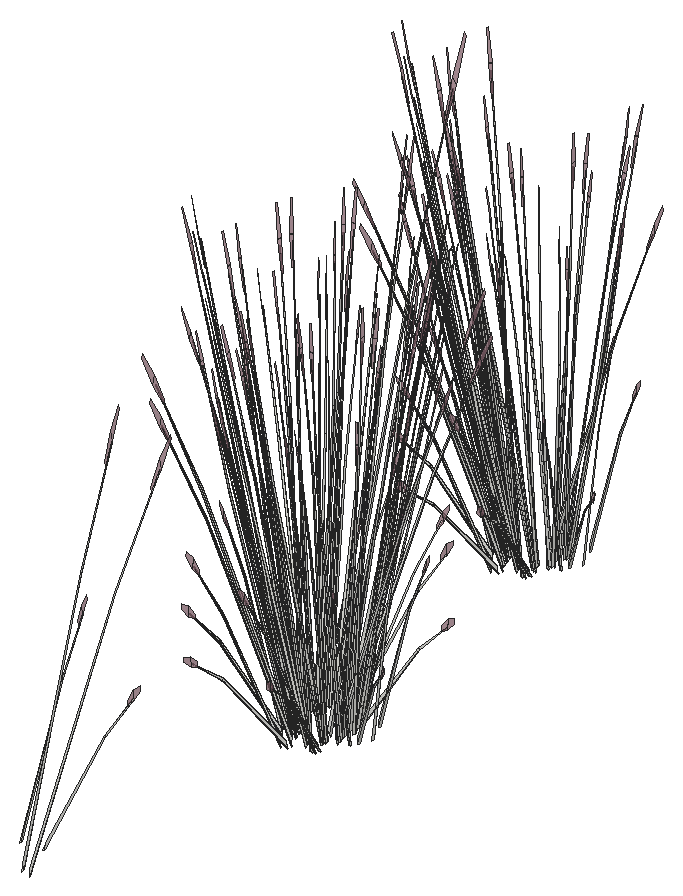
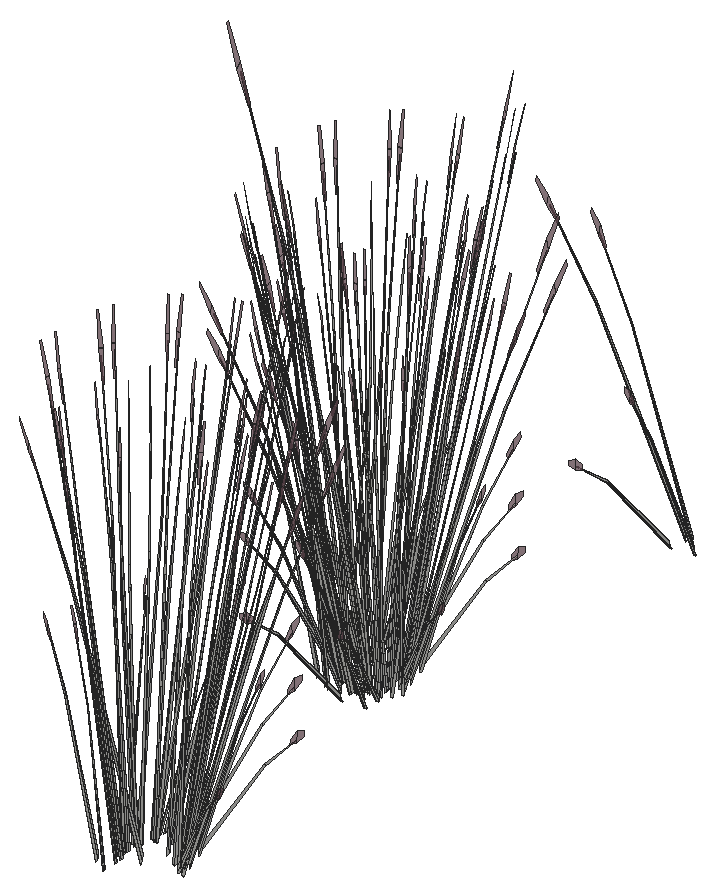
# SketchUp Ruby script. Lengths in inches.
U = 1.inch
M = Sketchup.active_model
def pt(a) = Geom::Point3d.new(a.map { |v| v * U })
def face(e, loops, mat)
  f = e.add_face(loops[0].map { |a| pt(a) })
  loops[1..].each { |l| e.add_face(l.map { |a| pt(a) }).erase! }
  f.material = f.back_material = mat if mat
  f
end
# faces: each face lists its corners as indices into pts; further lists are holes
def faces(e, pts, list, mat = nil) = list.each { |f| face(e, (f[0].is_a?(Array) ? f : [f]).map { |l| l.map { |i| pts[i] } }, mat) }
# xy, xz, yz: faces in a plane at the given z, y or x. An outline is a flat list of corners, or four numbers for a rectangle; further outlines are holes
def ring(l) = l.size == 4 ? [[l[0], l[1]], [l[2], l[1]], [l[2], l[3]], [l[0], l[3]]] : l.each_slice(2).to_a
def flat(e, list, mat, &to3) = list.each { |f| face(e, (f[0].is_a?(Array) ? f : [f]).map { |l| ring(l).map { |u, v| to3.(u, v) } }, mat) }
def xy(e, z, list, mat = nil) = flat(e, list, mat) { |x, y| [x, y, z] }
def xz(e, y, list, mat = nil) = flat(e, list, mat) { |x, z| [x, y, z] }
def yz(e, x, list, mat = nil) = flat(e, list, mat) { |y, z| [x, y, z] }
def lines(e, pts, list) = list.each { |a, b| e.add_line(pt(pts[a]), pt(pts[b])) }
# prism: a flat outline (further loops are holes) pulled along v
def prism(e, loops, v, mat = nil)
  f = face(e, loops, mat); d = Geom::Vector3d.new(v.map { |x| x * U })
  f.pushpull(f.normal.samedirection?(d) ? d.length : -d.length)
end
def box(e, o, s, mat = nil) = prism(e, [[o, [o[0] + s[0], o[1], o[2]], [o[0] + s[0], o[1] + s[1], o[2]], [o[0], o[1] + s[1], o[2]]]], [0, 0, s[2]], mat)
def at(x, y, z, deg = 0) = Geom::Transformation.translation(pt([x, y, z])) * Geom::Transformation.rotation(ORIGIN, Z_AXIS, deg.degrees)
def axes(o, x, y, z) = Geom::Transformation.new([*x, 0, *y, 0, *z, 0, *pt(o).to_a, 1])
def part(name) = M.definitions.add(name)
# library, detail: a bought-in or finely detailed component or shape, given as its bounding box
def library(name, o, s) = part(name).tap { |d| box(d.entities, o, s) }
def detail(e, o, s) = box(e.add_group.entities, o, s)
def put(e, d, t, mat = nil) = e.add_instance(d, t).tap { |i| i.material = mat if mat }
def group(e, t, mat = nil) = e.add_group.tap { |g| g.transformation = t; g.material = mat if mat }.entities
root = M.entities
M.materials.add("LightPink_Translucent").color = [144, 107, 117]
M.materials["LightPink_Translucent"].alpha = 0.75
c1 = part("blade")
p = [[2.15,0.21,22],[0,0.17,0],[0.09,0.45,0],[2.18,0.31,22],[2.29,0.31,22],[0.38,0.45,0],
  [2.48,0.24,33],[2.49,0.24,33],[2.48,0.22,33]]
faces(c1.entities,p,[[0,1,2,3],[4,5,2,3],[6,3,4,7],[8,0,3,6]])
c2 = part("seeds")
p = [[0.3,-0.1,1.38],[-0.01,-0.03,1.59],[-0.01,-0.03,0.03],[0.14,-0.07,-0.07],[0.29,-0.03,3],[0.15,0.01,3.11]]
faces(c2.entities,p,[[0,1,2,3],[1,0,4,5]],"LightPink_Translucent")
c3 = part("blade with seeds")
put(c3.entities,c1,at(0,0,0))
put(c3.entities,c2,axes([2.4,0.25,30.99],[1.5799,-0.05474,1.17369],[-0.12525,1.92788,0.29478],[-0.07173,-0.02425,1.56792]))
put(root,c3,axes([432.62,162.45,1.33],[-0.08601,-0.17716,1.47384],[0.39746,-0.14915,0.11917],[0.08983,0.27813,0.63005]))
put(root,c3,axes([430.45,164.24,2.05],[0.04269,-0.03331,1.5255],[0.35284,0.2216,-0.14414],[-0.00829,0.1845,0.26996]))
put(root,c3,axes([431.92,162.54,1.33],[-0.00921,-0.21179,1.47384],[0.39917,0.1405,0.11917],[-0.02469,0.30182,0.63005]))
put(root,c3,axes([432.01,164.47,2.05],[0.0477,0.08886,1.50452],[0.38493,0.03491,-0.23794],[0.03871,0.19596,0.12066]))
put(root,c3,axes([435.13,184.08,1.33],[0.08601,0.17716,1.47384],[-0.39746,0.14915,0.11917],[-0.08983,-0.27813,0.63005]))
put(root,c3,axes([435.79,182.9,2.05],[-0.05755,-0.07737,1.50452],[-0.38409,0.04905,-0.23794],[-0.0613,-0.18505,0.12066]))
put(root,c3,axes([437.51,183.85,2.05],[-0.00363,-0.10982,1.50452],[-0.30678,-0.3174,-0.23794],[0.04743,-0.1924,0.12066]))
put(root,c3,axes([436.22,183.83,1.89],[0.11344,-0.42434,-0.30456],[0.33096,0.12377,0.39319],[-0.03035,-0.17085,0.75234]))
put(root,c3,axes([436.47,184.39,1.33],[-0.07006,0.18966,1.47384],[-0.29392,-0.3925,0.11917],[0.13259,-0.24463,0.63005]))
put(root,c3,axes([437.43,183.46,2.05],[-0.03821,0.04215,1.5255],[-0.37441,-0.1422,-0.14414],[-0.01355,-0.18393,0.26996]))
put(root,c3,axes([435.39,182.65,2.05],[-0.00702,0.06614,1.5255],[-0.34622,0.24004,-0.14414],[-0.10188,-0.1227,0.26996]))
put(root,c3,axes([435.32,183.82,2.38],[0.41917,-0.14183,0.46236],[0.07275,0.55635,0.38124],[-0.09858,-0.16397,0.95674]))
put(root,c3,axes([436.26,183.93,2.07],[0.37078,0.14426,0.41282],[-0.12679,0.47426,0.34039],[-0.02228,-0.18651,0.85423]))
put(root,c3,axes([436.37,184.1,2.33],[-0.36822,0.25691,-0.10458],[-0.18095,-0.45596,-0.58045],[-0.04858,-0.19215,0.88199]))
put(root,c3,axes([437.14,184.67,2.33],[-0.41355,-0.02734,-0.10458],[0.0113,-0.51765,-0.58045],[0.02873,-0.19937,0.88199]))
put(root,c3,axes([436.36,183.89,2.07],[0.27727,-0.18753,0.0553],[0.13571,0.34197,0.43534],[-0.02678,-0.15075,0.66383]))
put(root,c3,axes([435.41,183.94,2.07],[0.17102,-0.35053,0.0553],[0.24354,0.20408,0.43534],[-0.07874,-0.11238,0.66383]))
put(root,c3,axes([434.55,184.63,1.33],[0.13977,0.09507,1.47384],[-0.28925,0.39884,0.11917],[-0.18028,-0.17992,0.63005]))
put(root,c3,axes([436.26,184.28,2.34],[-0.11344,0.42434,0.30456],[-0.33096,-0.12377,-0.39319],[-0.03035,-0.17085,0.75234]))
put(root,c3,axes([437.11,184.46,2.07],[0.26795,0.37649,0.41282],[-0.28456,0.3247,0.34039],[0.04943,-0.17664,0.85423]))
put(root,c3,axes([435.49,183.91,2.67],[-0.25113,0.52899,-0.11713],[-0.36369,-0.30476,-0.65011],[-0.12642,-0.14945,0.98783]))
put(root,c3,axes([437.21,184.49,2.07],[0.30922,0.02571,0.0553],[-0.00848,0.38824,0.43534],[0.03236,-0.14872,0.66383]))
put(root,c3,axes([436.97,184.75,2.34],[-0.2546,0.29052,0.30456],[-0.24101,-0.33173,-0.39319],[0.03667,-0.16855,0.75234]))
put(root,c3,axes([434.53,183.76,2.05],[-0.08096,-0.00389,1.50452],[-0.25776,0.38949,-0.23794],[-0.13753,-0.07958,0.12066]))
put(root,c3,axes([437.59,185.69,2.33],[-0.34807,-0.30426,-0.10458],[0.20053,-0.44063,-0.58045],[0.09834,-0.15317,0.88199]))
put(root,c3,axes([435.47,184.35,2.34],[0.05812,0.44446,0.30456],[-0.33222,0.11736,-0.39319],[-0.08923,-0.12737,0.75234]))
put(root,c3,axes([434.47,184.64,2.38],[0.31075,-0.40722,0.46236],[0.268,0.43246,0.38124],[-0.14579,-0.07512,0.95674]))
put(root,c3,axes([438.44,185.5625,2.05],[-0.04915,-0.00419,1.5255],[-0.20409,-0.44904,-0.14414],[0.08196,-0.14765,0.26996]))
put(root,c3,axes([434.61,184.63,2.07],[0.01895,-0.4196,0.0553],[0.28611,0.0115,0.43534],[-0.1096,-0.04391,0.66383]))
put(root,c3,axes([434.5,184.77,1.89],[-0.2141,-0.34548,-0.30456],[0.24447,-0.32704,0.39319],[-0.12421,-0.04976,0.75234]))
put(root,c3,axes([437.42,185.65,2.34],[-0.32754,0.07886,0.30456],[-0.08649,-0.45081,-0.39319],[0.09386,-0.12109,0.75234]))
put(root,c3,axes([437.71,185.58,2.07],[0.25832,0.23207,0.0553],[-0.1504,0.33047,0.43534],[0.08282,-0.10684,0.66383]))
put(root,c3,axes([437.64,185.48,2.07],[0.09332,0.50785,0.41282],[-0.36608,0.08814,0.34039],[0.10789,-0.11944,0.85423]))
put(root,c3,axes([438.63,186.1,2.05],[0.05222,-0.08405,1.50452],[-0.06683,-0.51557,-0.23794],[0.13101,-0.09775,0.12066]))
put(root,c3,axes([434.22,184.09,2.05],[0.0279,0.05507,1.5255],[-0.13448,0.49501,-0.14414],[-0.1362,0.00358,0.26996]))
put(root,c3,axes([434.8,184.95,2.34],[0.2141,0.34548,0.30456],[-0.24447,0.32704,-0.39319],[-0.12421,-0.04976,0.75234]))
put(root,c3,axes([434.75,184.73,2.33],[-0.02015,0.56117,-0.10458],[-0.38148,-0.01534,-0.58045],[-0.14692,-0.03898,0.88199]))
put(root,c3,axes([437.6,186.88,2.33],[-0.18933,-0.49965,-0.10458],[0.33602,-0.24554,-0.58045],[0.1416,-0.06592,0.88199]))
put(root,c3,axes([434.26,185.5,1.33],[0.15608,-0.0125,1.47384],[-0.10354,0.54165,0.11917],[-0.22242,-0.0335,0.63005]))
put(root,c3,axes([437.47,186.73,2.34],[-0.31272,-0.15393,0.30456],[0.09121,-0.44909,-0.39319],[0.1259,-0.04118,0.75234]))
put(root,c3,axes([434.2,185.91,2.07],[0.10631,-0.50312,0.41282],[0.34951,0.17204,0.34039],[-0.13745,0.03024,0.85423]))
put(root,c3,axes([434.17,185.78,2.07],[-0.1382,-0.37624,0.0553],[0.25202,-0.18416,0.43534],[-0.11109,0.03633,0.66383]))
put(root,c3,axes([436.95,186.125,1.33],[-0.15608,0.0125,1.47384],[0.10354,-0.54165,0.11917],[0.22242,0.0335,0.63005]))
put(root,c3,axes([437.75,186.87,2.07],[0.1382,0.37624,0.0553],[-0.25202,0.18416,0.43534],[0.11109,-0.03633,0.66383]))
put(root,c3,axes([437.73,186.74,2.07],[-0.10631,0.50312,0.41282],[-0.34951,-0.17204,0.34039],[0.13745,-0.03024,0.85423]))
put(root,c3,axes([434.45,185.92,2.34],[0.31272,0.15393,0.30456],[-0.09121,0.44909,-0.39319],[-0.1259,0.04118,0.75234]))
put(root,c3,axes([438.35,188.36,2.05],[-0.03403,-0.04831,1.5255],[0.07443,-0.51782,-0.14414],[0.13402,-0.03308,0.26996]))
put(root,c3,axes([433.93,186.26,2.05],[-0.06145,0.07164,1.50452],[0.00523,0.52344,-0.23794],[-0.14085,0.06807,0.12066]))
put(root,c3,axes([434.32,185.76,2.33],[0.18933,0.49965,-0.10458],[-0.33602,0.24554,-0.58045],[-0.1416,0.06592,0.88199]))
put(root,c3,axes([438.06,187.93,1.38],[-0.07202,-0.46385,-0.03003],[0.3404,-0.10664,-0.13615],[0.07108,0.02941,0.44908]))
put(root,c3,axes([437.18,187.92,2.33],[0.02015,-0.56117,-0.10458],[0.38148,0.01534,-0.58045],[0.14692,0.03898,0.88199]))
put(root,c3,axes([437.12,187.7,2.34],[-0.2141,-0.34548,0.30456],[0.24447,-0.32704,-0.39319],[0.12421,0.04976,0.75234]))
put(root,c3,axes([437.51,187.58,2.05],[0.08072,-0.00933,1.50452],[0.22141,-0.42869,-0.23794],[0.14358,0.05659,0.12066]))
put(root,c3,axes([434.28,187.16,2.07],[-0.09332,-0.50785,0.41282],[0.36608,-0.08814,0.34039],[-0.10789,0.11944,0.85423]))
put(root,c3,axes([434.21,187.07,2.07],[-0.25832,-0.23207,0.0553],[0.1504,-0.33047,0.43534],[-0.08282,0.10684,0.66383]))
put(root,c3,axes([434.32,186.45,1.33],[0.13056,-0.11672,1.47384],[0.10992,0.53933,0.11917],[-0.20497,0.12189,0.63005]))
put(root,c3,axes([434.5,186.99,2.34],[0.32754,-0.07886,0.30456],[0.08649,0.45081,-0.39319],[-0.09386,0.12109,0.75234]))
put(root,c3,axes([433.24,186.79,2.05],[0.04802,0.0148,1.5255],[0.14856,0.48754,-0.14414],[-0.0983,0.12796,0.26996]))
put(root,c3,axes([437.3125,188.01,2.07],[-0.01895,0.4196,0.0553],[-0.28611,-0.0115,0.43534],[0.1096,0.04391,0.66383]))
put(root,c3,axes([437.34,187.88,2.07],[-0.27746,0.36359,0.41282],[-0.23929,-0.38612,0.34039],[0.13017,0.06707,0.85423]))
put(root,c3,axes([433.76,188.27,2.86],[0.33205,0.14729,-0.05579],[-0.10214,0.45334,-0.25298],[-0.05431,0.06883,0.83441]))
put(root,c3,axes([436.45,188.3,2.34],[-0.05812,-0.44446,0.30456],[0.33222,-0.11736,-0.39319],[0.08923,0.12737,0.75234]))
put(root,c3,axes([436.65,186.99,1.33],[-0.13977,-0.09507,1.47384],[0.28925,-0.39884,0.11917],[0.18028,0.17992,0.63005]))
put(root,c3,axes([436.68,185.74,1.85],[-0.32515,-0.2867,1.18923],[0.34333,-0.44639,0.51312],[0.10491,0.26901,1.1495]))
put(root,c3,axes([434.33,186.95,2.33],[0.34807,0.30426,-0.10458],[-0.20053,0.44063,-0.58045],[-0.09834,0.15317,0.88199]))
put(root,c3,axes([436.42,188.53,2.33],[0.22423,-0.47232,-0.10458],[0.32472,0.27211,-0.58045],[0.11288,0.13344,0.88199]))
put(root,c3,axes([434.8,186.82,1.33],[0.09398,-0.16955,1.47384],[0.23731,0.45764,0.11917],[-0.16276,0.20841,0.63005]))
put(root,c3,axes([434.95,187.89,2.34],[0.2546,-0.29052,0.30456],[0.24101,0.33173,-0.39319],[-0.03667,0.16855,0.75234]))
put(root,c3,axes([436.13,188.92,2.05],[0.00111,-0.06681,1.5255],[0.32247,-0.29474,-0.14414],[0.11201,0.1052,0.26996]))
put(root,c3,axes([434.72,188.16,2.07],[-0.30922,-0.02571,0.0553],[0.00848,-0.38824,0.43534],[-0.03236,0.14872,0.66383]))
put(root,c3,axes([434.8125,188.19,2.07],[-0.26795,-0.37649,0.41282],[0.28456,-0.3247,0.34039],[-0.04943,0.17664,0.85423]))
put(root,c3,axes([435.66,188.37,2.34],[0.11344,-0.42434,0.30456],[0.33096,0.12377,-0.39319],[0.03035,0.17085,0.75234]))
put(root,c3,axes([436.51,188.7,2.07],[-0.17102,0.35053,0.0553],[-0.24354,-0.20408,0.43534],[0.07874,0.11238,0.66383]))
put(root,c3,axes([436.11,189.88,2.86],[0.26003,-0.31656,-0.05579],[0.23826,0.3467,-0.25298],[0.01677,0.09824,0.83441]))
put(root,c3,axes([436.58,188.6,2.07],[-0.37426,0.12663,0.41282],[-0.06495,-0.49674,0.34039],[0.08802,0.1464,0.85423]))
put(root,c3,axes([434.73,187.23,1.33],[0.07006,-0.18966,1.47384],[0.29392,0.3925,0.11917],[-0.13259,0.24463,0.63005]))
put(root,c3,axes([435.56,188.75,2.07],[-0.27727,0.18753,0.0553],[-0.13571,-0.34197,0.43534],[0.02678,0.15075,0.66383]))
put(root,c3,axes([433.94,188.22,2.05],[-0.00935,0.1092,1.50452],[0.26544,0.37987,-0.23794],[-0.06949,0.17964,0.12066]))
put(root,c3,axes([434.78,187.97,2.64],[0.41355,0.02734,-0.11608],[-0.0113,0.51765,-0.6443],[-0.02873,0.19937,0.97901]))
put(root,c3,axes([435.55,188.55,2.33],[0.36822,-0.25691,-0.10458],[0.18095,0.45596,-0.58045],[0.04858,0.19215,0.88199]))
put(root,c3,axes([435.66,188.72,2.35],[-0.37078,-0.14426,0.45823],[0.12679,-0.47426,0.37783],[0.02228,0.18651,0.9482]))
put(root,c3,axes([436.08,187.55,1.33],[-0.08601,-0.17716,1.47384],[0.39746,-0.14915,0.11917],[0.08983,0.27813,0.63005]))
put(root,c3,axes([433.91,189.34,2.05],[0.04269,-0.03331,1.5255],[0.35284,0.2216,-0.14414],[-0.00829,0.1845,0.26996]))
put(root,c3,axes([435.37,187.63,1.33],[-0.00921,-0.21179,1.47384],[0.39917,0.1405,0.11917],[-0.02469,0.30182,0.63005]))
put(root,c3,axes([435.46,189.57,2.05],[0.0477,0.08886,1.50452],[0.38493,0.03491,-0.23794],[0.03871,0.19596,0.12066]))
put(root,c3,axes([431.68,208.18,1.33],[0.08601,0.17716,1.47384],[-0.39746,0.14915,0.11917],[-0.08983,-0.27813,0.63005]))
put(root,c3,axes([432.33,207,2.05],[-0.05755,-0.07737,1.50452],[-0.38409,0.04905,-0.23794],[-0.0613,-0.18505,0.12066]))
put(root,c3,axes([434.06,207.95,2.05],[-0.00363,-0.10982,1.50452],[-0.30678,-0.3174,-0.23794],[0.04743,-0.1924,0.12066]))
put(root,c3,axes([432.77,207.93,1.89],[0.11344,-0.42434,-0.30456],[0.33096,0.12377,0.39319],[-0.03035,-0.17085,0.75234]))
put(root,c3,axes([433.02,208.49,1.33],[-0.07006,0.18966,1.47384],[-0.29392,-0.3925,0.11917],[0.13259,-0.24463,0.63005]))
put(root,c3,axes([433.98,207.55,2.05],[-0.03821,0.04215,1.5255],[-0.37441,-0.1422,-0.14414],[-0.01355,-0.18393,0.26996]))
put(root,c3,axes([431.9375,206.75,2.05],[-0.00702,0.06614,1.5255],[-0.34622,0.24004,-0.14414],[-0.10188,-0.1227,0.26996]))
put(root,c3,axes([431.86,207.92,2.38],[0.41917,-0.14183,0.46236],[0.07275,0.55635,0.38124],[-0.09858,-0.16397,0.95674]))
put(root,c3,axes([432.81,208.02,2.07],[0.37078,0.14426,0.41282],[-0.12679,0.47426,0.34039],[-0.02228,-0.18651,0.85423]))
put(root,c3,axes([432.92,208.19,2.33],[-0.36822,0.25691,-0.10458],[-0.18095,-0.45596,-0.58045],[-0.04858,-0.19215,0.88199]))
put(root,c3,axes([433.68,208.77,2.33],[-0.41355,-0.02734,-0.10458],[0.0113,-0.51765,-0.58045],[0.02873,-0.19937,0.88199]))
put(root,c3,axes([433.65,208.4375,1.89],[0.2546,-0.29052,-0.30456],[0.24101,0.33173,0.39319],[0.03667,-0.16855,0.75234]))
put(root,c3,axes([432.91,207.99,2.07],[0.27727,-0.18753,0.0553],[0.13571,0.34197,0.43534],[-0.02678,-0.15075,0.66383]))
put(root,c3,axes([431.82,208.08,1.89],[-0.05812,-0.44446,-0.30456],[0.33222,-0.11736,0.39319],[-0.08923,-0.12737,0.75234]))
put(root,c3,axes([431.96,208.04,2.07],[0.17102,-0.35053,0.0553],[0.24354,0.20408,0.43534],[-0.07874,-0.11238,0.66383]))
put(root,c3,axes([431.1,208.73,1.33],[0.13977,0.09507,1.47384],[-0.28925,0.39884,0.11917],[-0.18028,-0.17992,0.63005]))
put(root,c3,axes([432.81,208.375,2.34],[-0.11344,0.42434,0.30456],[-0.33096,-0.12377,-0.39319],[-0.03035,-0.17085,0.75234]))
put(root,c3,axes([433.65,208.55,2.07],[0.26795,0.37649,0.41282],[-0.28456,0.3247,0.34039],[0.04943,-0.17664,0.85423]))
put(root,c3,axes([432.04,208,2.67],[-0.25113,0.52899,-0.11713],[-0.36369,-0.30476,-0.65011],[-0.12642,-0.14945,0.98783]))
put(root,c3,axes([433.75,208.59,2.07],[0.30922,0.02571,0.0553],[-0.00848,0.38824,0.43534],[0.03236,-0.14872,0.66383]))
put(root,c3,axes([433.52,208.85,2.34],[-0.2546,0.29052,0.30456],[-0.24101,-0.33173,-0.39319],[0.03667,-0.16855,0.75234]))
put(root,c3,axes([431.07,207.85,2.05],[-0.08096,-0.00389,1.50452],[-0.25776,0.38949,-0.23794],[-0.13753,-0.07958,0.12066]))
put(root,c3,axes([434.13,209.79,2.33],[-0.34807,-0.30426,-0.10458],[0.20053,-0.44063,-0.58045],[0.09834,-0.15317,0.88199]))
put(root,c3,axes([432.01,208.44,2.34],[0.05812,0.44446,0.30456],[-0.33222,0.11736,-0.39319],[-0.08923,-0.12737,0.75234]))
put(root,c3,axes([431.01,208.73,2.38],[0.31075,-0.40722,0.46236],[0.268,0.43246,0.38124],[-0.14579,-0.07512,0.95674]))
put(root,c3,axes([434.99,209.66,2.05],[-0.04915,-0.00419,1.5255],[-0.20409,-0.44904,-0.14414],[0.08196,-0.14765,0.26996]))
put(root,c3,axes([434.23,209.48,1.89],[0.32754,-0.07886,-0.30456],[0.08649,0.45081,0.39319],[0.09386,-0.12109,0.75234]))
put(root,c3,axes([431.16,208.73,2.07],[0.01895,-0.4196,0.0553],[0.28611,0.0115,0.43534],[-0.1096,-0.04391,0.66383]))
put(root,c3,axes([431.05,208.86,1.89],[-0.2141,-0.34548,-0.30456],[0.24447,-0.32704,0.39319],[-0.12421,-0.04976,0.75234]))
put(root,c3,axes([433.96,209.75,2.34],[-0.32754,0.07886,0.30456],[-0.08649,-0.45081,-0.39319],[0.09386,-0.12109,0.75234]))
put(root,c3,axes([434.26,209.68,2.07],[0.25832,0.23207,0.0553],[-0.1504,0.33047,0.43534],[0.08282,-0.10684,0.66383]))
put(root,c3,axes([434.1875,209.58,2.07],[0.09332,0.50785,0.41282],[-0.36608,0.08814,0.34039],[0.10789,-0.11944,0.85423]))
put(root,c3,axes([435.17,210.2,2.05],[0.05222,-0.08405,1.50452],[-0.06683,-0.51557,-0.23794],[0.13101,-0.09775,0.12066]))
put(root,c3,axes([430.76,208.18,2.05],[0.0279,0.05507,1.5255],[-0.13448,0.49501,-0.14414],[-0.1362,0.00358,0.26996]))
put(root,c3,axes([431.35,209.04,2.34],[0.2141,0.34548,0.30456],[-0.24447,0.32704,-0.39319],[-0.12421,-0.04976,0.75234]))
put(root,c3,axes([431.29,208.82,2.33],[-0.02015,0.56117,-0.10458],[-0.38148,-0.01534,-0.58045],[-0.14692,-0.03898,0.88199]))
put(root,c3,axes([434.15,210.98,2.33],[-0.18933,-0.49965,-0.10458],[0.33602,-0.24554,-0.58045],[0.1416,-0.06592,0.88199]))
put(root,c3,axes([430.81,209.6,1.33],[0.15608,-0.0125,1.47384],[-0.10354,0.54165,0.11917],[-0.22242,-0.0335,0.63005]))
put(root,c3,axes([434.01,210.83,2.34],[-0.31272,-0.15393,0.30456],[0.09121,-0.44909,-0.39319],[0.1259,-0.04118,0.75234]))
put(root,c3,axes([430.74,210.01,2.07],[0.10631,-0.50312,0.41282],[0.34951,0.17204,0.34039],[-0.13745,0.03024,0.85423]))
put(root,c3,axes([430.71,209.875,2.07],[-0.1382,-0.37624,0.0553],[0.25202,-0.18416,0.43534],[-0.11109,0.03633,0.66383]))
put(root,c3,axes([434.34,210.78,1.89],[0.31272,0.15393,-0.30456],[-0.09121,0.44909,0.39319],[0.1259,-0.04118,0.75234]))
put(root,c3,axes([430.67,210.0625,1.89],[-0.31272,-0.15393,-0.30456],[0.09121,-0.44909,0.39319],[-0.1259,0.04118,0.75234]))
put(root,c3,axes([433.49,210.22,1.33],[-0.15608,0.0125,1.47384],[0.10354,-0.54165,0.11917],[0.22242,0.0335,0.63005]))
put(root,c3,axes([434.3,210.97,2.07],[0.1382,0.37624,0.0553],[-0.25202,0.18416,0.43534],[0.11109,-0.03633,0.66383]))
put(root,c3,axes([434.27,210.83,2.07],[-0.10631,0.50312,0.41282],[-0.34951,-0.17204,0.34039],[0.13745,-0.03024,0.85423]))
put(root,c3,axes([431,210.01,2.34],[0.31272,0.15393,0.30456],[-0.09121,0.44909,-0.39319],[-0.1259,0.04118,0.75234]))
put(root,c3,axes([434.9,212.46,2.05],[-0.03403,-0.04831,1.5255],[0.07443,-0.51782,-0.14414],[0.13402,-0.03308,0.26996]))
put(root,c3,axes([430.47,210.36,2.05],[-0.06145,0.07164,1.50452],[0.00523,0.52344,-0.23794],[-0.14085,0.06807,0.12066]))
put(root,c3,axes([430.87,209.86,2.33],[0.18933,0.49965,-0.10458],[-0.33602,0.24554,-0.58045],[-0.1416,0.06592,0.88199]))
put(root,c3,axes([434.6,212.03,1.38],[-0.07202,-0.46385,-0.03003],[0.3404,-0.10664,-0.13615],[0.07108,0.02941,0.44908]))
put(root,c3,axes([433.72,212.02,2.33],[0.02015,-0.56117,-0.10458],[0.38148,0.01534,-0.58045],[0.14692,0.03898,0.88199]))
put(root,c3,axes([433.66,211.8,2.34],[-0.2141,-0.34548,0.30456],[0.24447,-0.32704,-0.39319],[0.12421,0.04976,0.75234]))
